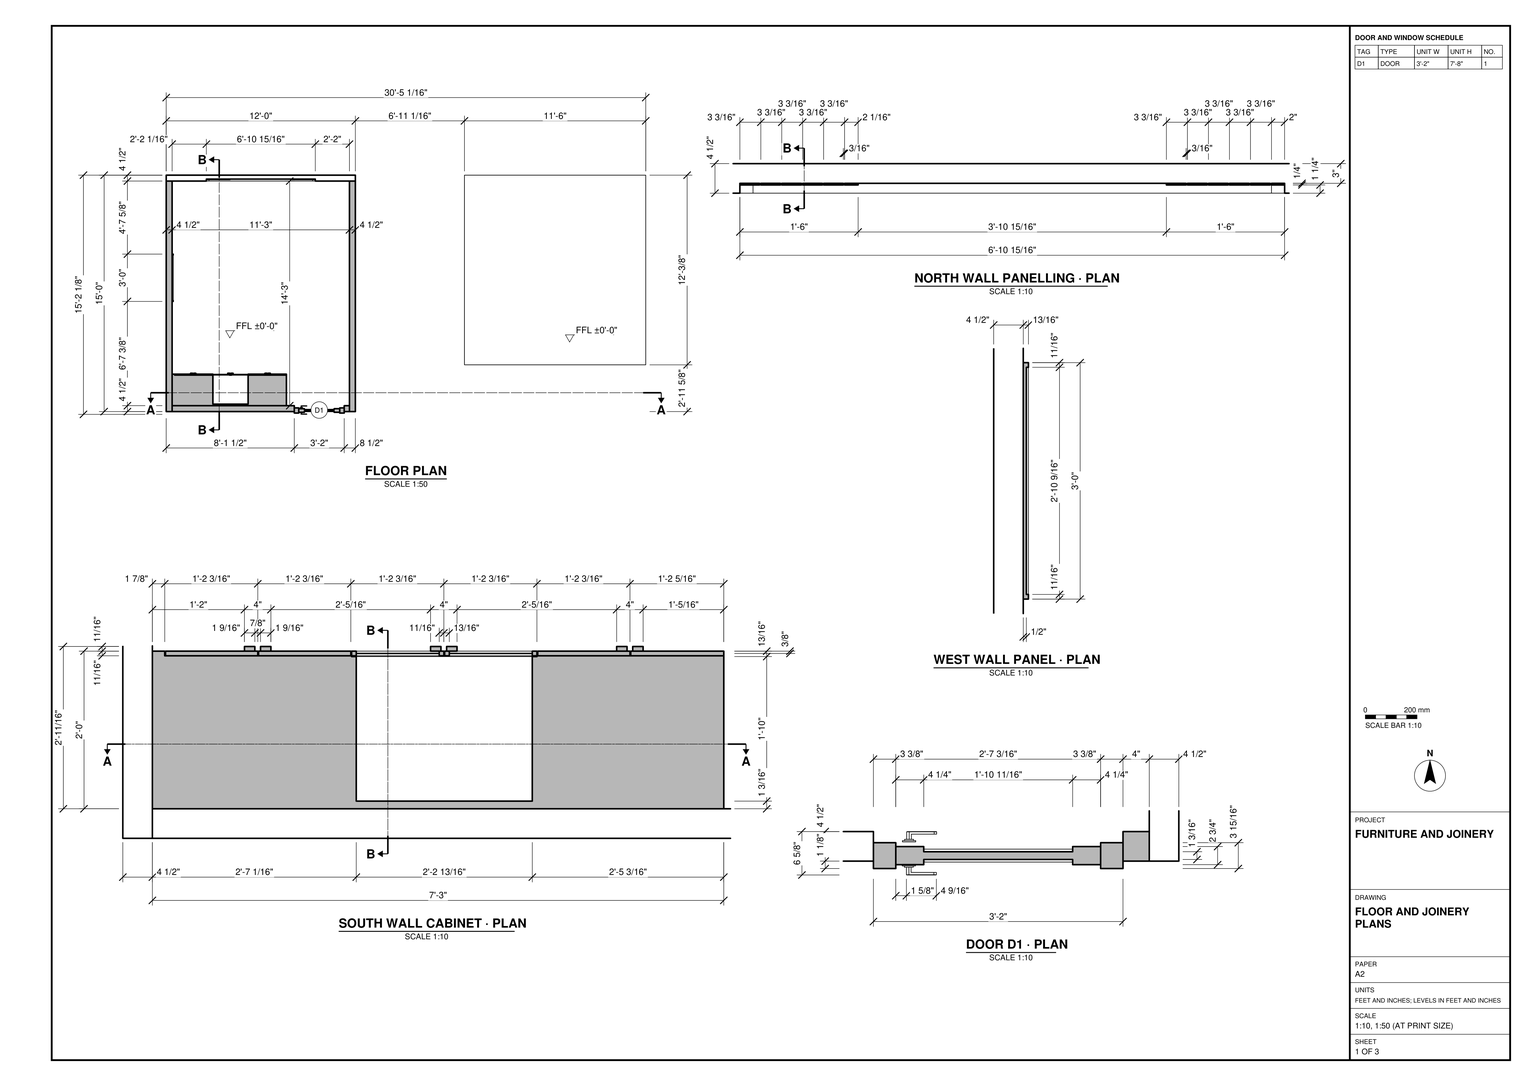
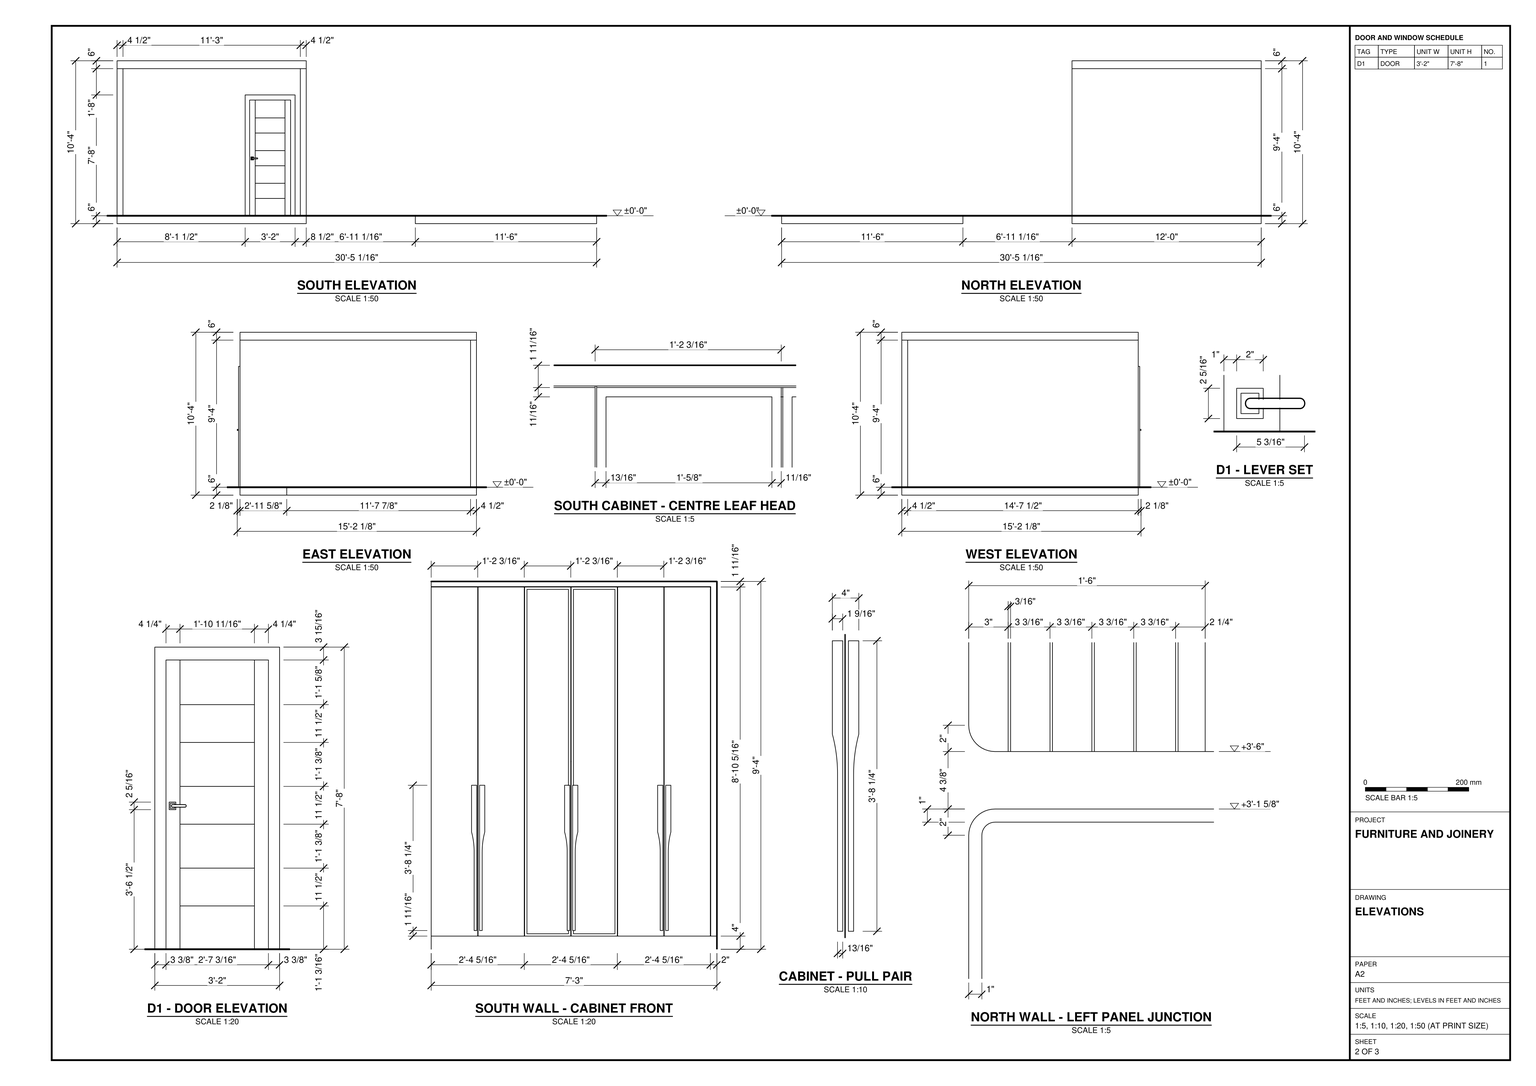
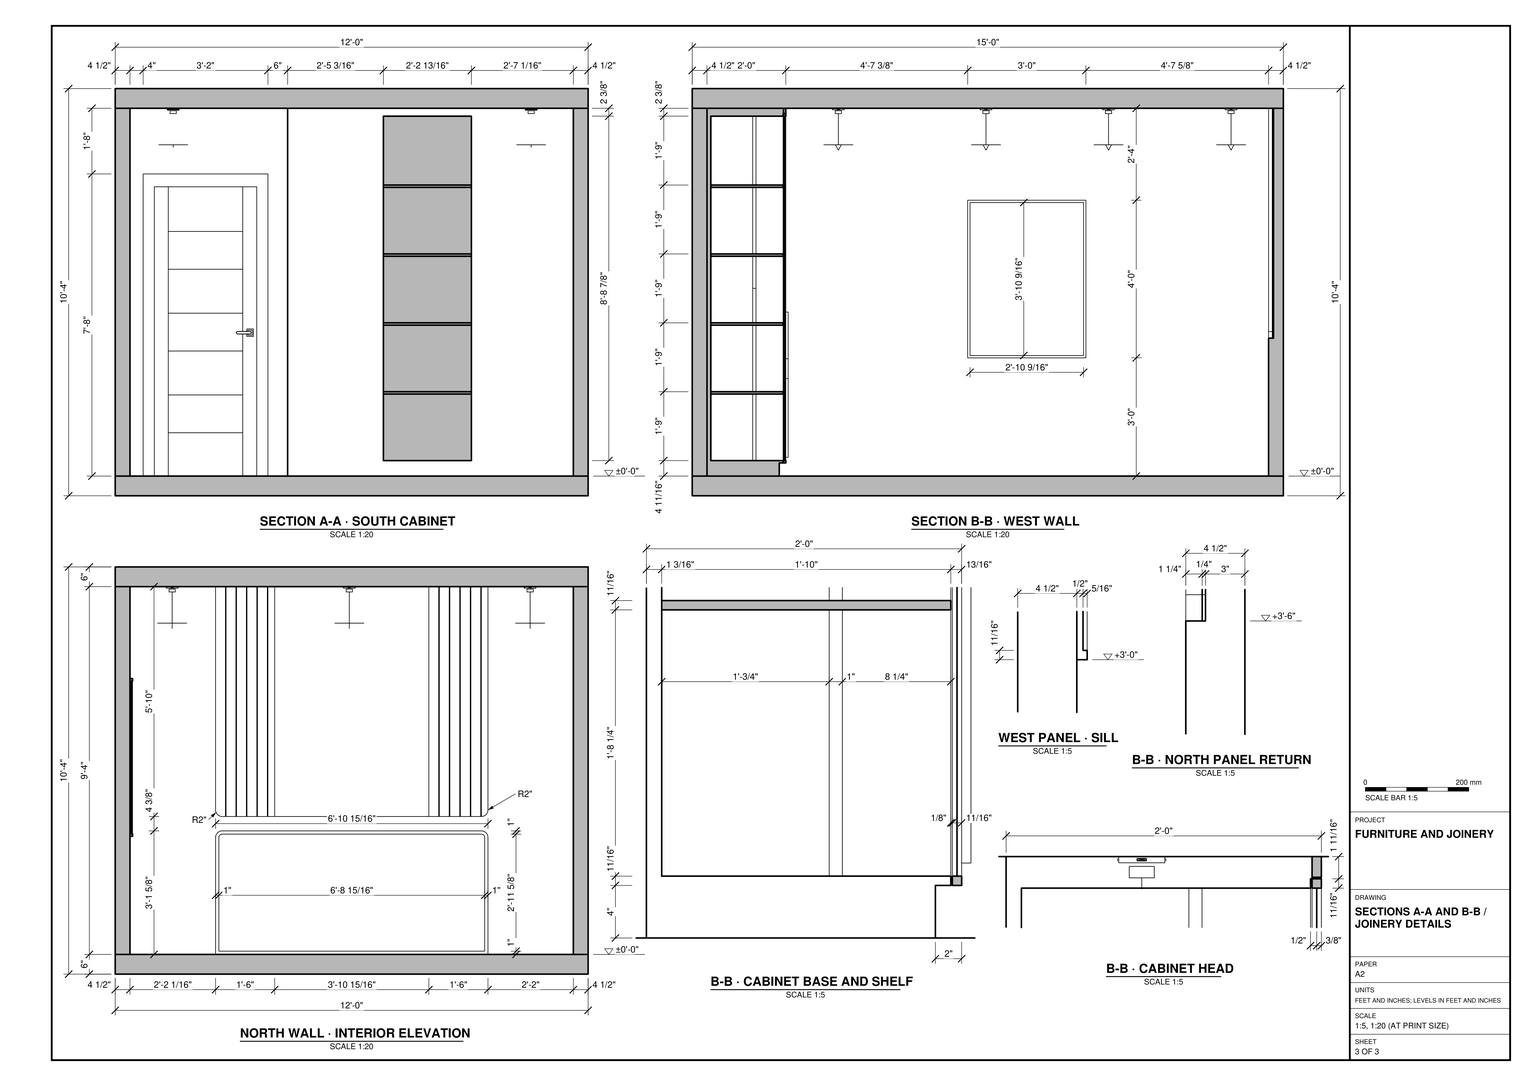
Build the room and its fitted joinery in SketchUp from task_files/diagram_01.pdf. Work in feet and inches. The complete layout is 30'-5 1/16" east to west by 15'-2 1/8" north to south, with an overall height of 10'-4". Use ±0'-0" as the finished floor level for both the room and the separate rectangular slab to its east. Keep the gap between them shown on the floor plan.

Form the room with 4 1/2" walls, a floor slab and a flat ceiling slab. Fit the framed door near the east end of the south wall, with the horizontal divisions and lever shown in elevation. Fit the full-height cabinet to the west of the door. Use the cabinet front and sections together to model the paired leaves, framed centre leaves, long pulls, shelves and recessed base.

On the north wall, model the lower framed panel and the upper panel with vertical divisions at its ends. Preserve the gap and rounded corners at their junction. On the west wall, fit the rectangular panel with its projecting sill. Place the ceiling lights as shown in section. Decor and loose items may be any suitable library components. Make the shell elements and each furniture or joinery piece separate groups or components, and use components for repeated parts. Save one SketchUp model as output_files/room_with_a_fitted_cabinet_and_wall_panelling.skp.

# SketchUp Ruby script. Lengths in inches.
U = 1.inch
M = Sketchup.active_model
def pt(a) = Geom::Point3d.new(a.map { |v| v * U })
def face(e, loops, mat)
  f = e.add_face(loops[0].map { |a| pt(a) })
  loops[1..].each { |l| e.add_face(l.map { |a| pt(a) }).erase! }
  f.material = f.back_material = mat if mat
  f
end
# faces: each face lists its corners as indices into pts; further lists are holes
def faces(e, pts, list, mat = nil) = list.each { |f| face(e, (f[0].is_a?(Array) ? f : [f]).map { |l| l.map { |i| pts[i] } }, mat) }
# xy, xz, yz: faces in a plane at the given z, y or x. An outline is a flat list of corners, or four numbers for a rectangle; further outlines are holes
def ring(l) = l.size == 4 ? [[l[0], l[1]], [l[2], l[1]], [l[2], l[3]], [l[0], l[3]]] : l.each_slice(2).to_a
def flat(e, list, mat, &to3) = list.each { |f| face(e, (f[0].is_a?(Array) ? f : [f]).map { |l| ring(l).map { |u, v| to3.(u, v) } }, mat) }
def xy(e, z, list, mat = nil) = flat(e, list, mat) { |x, y| [x, y, z] }
def xz(e, y, list, mat = nil) = flat(e, list, mat) { |x, z| [x, y, z] }
def yz(e, x, list, mat = nil) = flat(e, list, mat) { |y, z| [x, y, z] }
def lines(e, pts, list) = list.each { |a, b| e.add_line(pt(pts[a]), pt(pts[b])) }
# prism: a flat outline (further loops are holes) pulled along v
def prism(e, loops, v, mat = nil)
  f = face(e, loops, mat); d = Geom::Vector3d.new(v.map { |x| x * U })
  f.pushpull(f.normal.samedirection?(d) ? d.length : -d.length)
end
def box(e, o, s, mat = nil) = prism(e, [[o, [o[0] + s[0], o[1], o[2]], [o[0] + s[0], o[1] + s[1], o[2]], [o[0], o[1] + s[1], o[2]]]], [0, 0, s[2]], mat)
def at(x, y, z, deg = 0) = Geom::Transformation.translation(pt([x, y, z])) * Geom::Transformation.rotation(ORIGIN, Z_AXIS, deg.degrees)
def axes(o, x, y, z) = Geom::Transformation.new([*x, 0, *y, 0, *z, 0, *pt(o).to_a, 1])
def part(name) = M.definitions.add(name)
# library, detail: a bought-in or finely detailed component or shape, given as its bounding box
def library(name, o, s) = part(name).tap { |d| box(d.entities, o, s) }
def detail(e, o, s) = box(e.add_group.entities, o, s)
def put(e, d, t, mat = nil) = e.add_instance(d, t).tap { |i| i.material = mat if mat }
def group(e, t, mat = nil) = e.add_group.tap { |g| g.transformation = t; g.material = mat if mat }.entities
root = M.entities
M.materials.add("0897 AP 7835 CREAM CARESS").color = [247, 240, 216]
M.materials.add("2106173_041").color = [3, 2, 0]
M.materials.add("[Color A07]").color = [153, 0, 0]
M.materials.add("[Color M00]").color = [255, 255, 255]
M.materials.add("[Color M09]").color = [0, 0, 0]
M.materials.add("[Translucent Glass Gray]").color = [128, 128, 128]
M.materials["[Translucent Glass Gray]"].alpha = 0.5
M.materials.add("lz-doorbrown").color = [51, 28, 20]
M.materials.add("lz-doorhandle").color = [114, 114, 114]
c1 = part("Door lever handle")
xy(c1.entities,0,[[0,0,1.888,1.971]])
xy(c1.entities,0.197,[[[0,0,1.888,1.971],[0.307,0.321,1.58,1.65]]])
xy(c1.entities,0.394,[[[0.307,0.321,1.58,1.65],[0.954,0.632,0.96,0.632,0.96,1.339,0.954,1.339,0.868,1.328,0.782,1.292,0.709,1.236,0.653,1.162,0.617,1.077,0.605,0.985,0.617,0.894,0.653,0.808,0.709,0.735,0.782,0.678,0.868,0.643]],[0.954,0.632,0.868,0.643,0.782,0.678,0.709,0.735,0.653,0.808,0.617,0.894,0.605,0.985,0.617,1.077,0.653,1.162,0.709,1.236,0.782,1.292,0.868,1.328,0.954,1.339,0.96,1.339,0.96,0.632],[0.96,0.632,1.265,1.339]])
xy(c1.entities,1.181,[[1.265,0.632,1.265,1.339,4.506,1.339,4.592,1.328,4.677,1.292,4.751,1.236,4.807,1.162,4.842,1.077,4.854,0.985,4.842,0.894,4.807,0.808,4.751,0.735,4.677,0.678,4.592,0.643,4.506,0.632]])
xy(c1.entities,1.535,[[0.954,0.632,0.868,0.643,0.782,0.678,0.709,0.735,0.653,0.808,0.617,0.894,0.605,0.985,0.617,1.077,0.653,1.162,0.709,1.236,0.782,1.292,0.868,1.328,0.954,1.339,4.506,1.339,4.592,1.328,4.677,1.292,4.751,1.236,4.807,1.162,4.842,1.077,4.854,0.985,4.842,0.894,4.807,0.808,4.751,0.735,4.677,0.678,4.592,0.643,4.506,0.632]])
xy(c1.entities,1.575,[[0.956,0.671,0.878,0.681,0.802,0.713,0.737,0.763,0.687,0.828,0.656,0.904,0.645,0.985,0.656,1.067,0.687,1.143,0.737,1.208,0.802,1.258,0.878,1.289,0.956,1.3,4.503,1.3,4.581,1.289,4.657,1.258,4.722,1.208,4.772,1.143,4.804,1.067,4.815,0.985,4.804,0.904,4.772,0.828,4.722,0.763,4.657,0.713,4.581,0.681,4.503,0.671]])
xz(c1.entities,0,[[0,0,1.888,0.197]])
xz(c1.entities,0.321,[[0.307,0.197,1.58,0.394]])
xz(c1.entities,0.632,[[0.954,0.394,0.96,1.535],[0.96,0.394,0.96,1.535,4.506,1.535,4.506,1.181,1.265,1.181,1.265,0.394]])
xz(c1.entities,1.339,[[0.954,0.394,0.96,1.535],[0.96,0.394,1.265,0.394,1.265,1.181,4.506,1.181,4.506,1.535,0.96,1.535]])
xz(c1.entities,1.65,[[0.307,0.197,1.58,0.394]])
xz(c1.entities,1.971,[[0,0,1.888,0.197]])
yz(c1.entities,0,[[0,0,1.971,0.197]])
yz(c1.entities,0.307,[[0.321,0.197,1.65,0.394]])
yz(c1.entities,1.265,[[0.632,0.394,1.339,1.181]])
yz(c1.entities,1.58,[[0.321,0.197,1.65,0.394]])
yz(c1.entities,1.888,[[0,0,1.971,0.197]])
p = [[0.782,0.678,1.535],[0.868,0.643,1.535],[0.868,0.643,0.394],[0.782,0.678,0.394],[0.954,0.632,1.535],[0.954,0.632,0.394],
  [0.653,0.808,1.535],[0.709,0.735,1.535],[0.709,0.735,0.394],[0.653,0.808,0.394],[0.617,0.894,1.535],[0.617,0.894,0.394],
  [0.605,0.985,1.535],[0.605,0.985,0.394],[0.617,1.077,1.535],[0.617,1.077,0.394],[0.653,1.162,1.535],[0.653,1.162,0.394],
  [0.782,1.292,1.535],[0.709,1.236,1.535],[0.709,1.236,0.394],[0.782,1.292,0.394],[0.868,1.328,1.535],[0.868,1.328,0.394],
  [0.954,1.339,1.535],[0.954,1.339,0.394],[4.592,0.643,1.535],[4.506,0.632,1.535],[4.506,0.632,1.181],[4.592,0.643,1.181],
  [4.677,0.678,1.535],[4.677,0.678,1.181],[4.751,0.735,1.535],[4.751,0.735,1.181],[4.807,0.808,1.535],[4.807,0.808,1.181],
  [4.842,0.894,1.535],[4.842,0.894,1.181],[4.854,0.985,1.535],[4.854,0.985,1.181],[4.842,1.077,1.535],[4.842,1.077,1.181],
  [4.807,1.162,1.535],[4.807,1.162,1.181],[4.677,1.292,1.535],[4.751,1.236,1.535],[4.751,1.236,1.181],[4.677,1.292,1.181],
  [4.506,1.339,1.535],[4.592,1.328,1.535],[4.592,1.328,1.181],[4.506,1.339,1.181],[0.802,0.713,1.575],[0.878,0.681,1.575],
  [0.956,0.671,1.575],[0.96,0.632,1.535],[0.96,0.671,1.575],[4.503,0.671,1.575],[4.581,0.681,1.575],[4.657,0.713,1.575],
  [0.687,0.828,1.575],[0.737,0.763,1.575],[4.722,0.763,1.575],[4.772,0.828,1.575],[0.656,0.904,1.575],[4.804,0.904,1.575],
  [0.645,0.985,1.575],[4.815,0.985,1.575],[0.656,1.067,1.575],[4.804,1.067,1.575],[0.687,1.143,1.575],[0.737,1.208,1.575],
  [4.772,1.143,1.575],[4.722,1.208,1.575],[0.802,1.258,1.575],[4.657,1.258,1.575],[0.878,1.289,1.575],[0.956,1.3,1.575],
  [0.96,1.3,1.575],[0.96,1.339,1.535],[4.503,1.3,1.575],[4.581,1.289,1.575]]
faces(c1.entities,p,[[0,1,2,3],[1,4,5,2],[6,7,8,9],[7,0,3,8],[10,6,9,11],[12,10,11,13],[14,12,13,15],[16,14,15,17],
  [18,19,20,21],[19,16,17,20],[22,18,21,23],[24,22,23,25],[26,27,28,29],[30,26,29,31],[32,30,31,33],[34,32,33,35],
  [36,34,35,37],[38,36,37,39],[40,38,39,41],[42,40,41,43],[44,45,46,47],[45,42,43,46],[48,49,50,51],[49,44,47,50],
  [0,52,53,1],[1,53,54,4],[55,56,57,27],[54,56,55,4],[27,57,58,26],[26,58,59,30],[6,60,61,7],[7,61,52,0],
  [30,59,62,32],[32,62,63,34],[10,64,60,6],[34,63,65,36],[12,66,64,10],[36,65,67,38],[14,68,66,12],[38,67,69,40],
  [16,70,68,14],[19,71,70,16],[42,72,73,45],[40,69,72,42],[18,74,71,19],[45,73,75,44],[22,76,74,18],[24,77,76,22],
  [78,77,24,79],[79,48,80,78],[49,81,80,48],[44,75,81,49]])
c2 = part("door by lz")
put(c2.entities,c1,axes([9.99,-3.35,36.38],[1,0,0],[0,0,1],[0,-1,0]),"lz-doorhandle")
put(c2.entities,c1,axes([10.03,0.12,36.38],[1,0,0],[0,0,1],[0,1,0]),"lz-doorhandle")
g1 = group(c2.entities,at(5.91,0,0),"lz-doorbrown")
prism(g1,[[[35.43,0,0],[32.26,0,0],[32.26,0,75.4],[3.18,0,75.4],[3.18,0,0],[0,0,0],[0,0,78.74],[35.43,0,78.74]]],[0,-3.9375,0])
g2 = group(c2.entities,at(9.09,-0.59,0),"lz-doorbrown")
xy(g2,0,[[0,-2.76,3.97,-2.76,3.97,-2.36,25.11,-2.36,25.11,-2.76,29.08,-2.76,29.08,0,25.11,0,25.11,-0.39,3.97,-0.39,3.97,0,0,0]])
xy(g2,11.29,[[3.97,-2.36,25.11,-1.97],[3.97,-0.79,25.11,-0.39]])
xy(g2,21.14,[[3.97,-2.36,25.11,-1.97],[3.97,-0.79,25.11,-0.39]])
xy(g2,32.6,[[3.97,-2.36,25.11,-1.97],[3.97,-0.79,25.11,-0.39]])
xy(g2,42.45,[[3.97,-2.36,25.11,-1.97],[3.97,-0.79,25.11,-0.39]])
xy(g2,53.9,[[3.97,-2.36,25.11,-1.97],[3.97,-0.79,25.11,-0.39]])
xy(g2,63.75,[[3.97,-2.36,25.11,-1.97],[3.97,-0.79,25.11,-0.39]])
xy(g2,75.4,[[0,-2.76,0,0,3.97,0,3.97,-0.39,25.11,-0.39,25.11,0,29.08,0,29.08,-2.76,25.11,-2.76,25.11,-2.36,3.97,-2.36,3.97,-2.76]])
xz(g2,-2.76,[[0,0,3.97,75.4],[25.11,0,29.08,75.4]])
xz(g2,-2.36,[[3.97,0,25.11,11.29],[3.97,21.14,25.11,32.6],[3.97,42.45,25.11,53.9],[3.97,63.75,25.11,75.4]])
xz(g2,-1.97,[[3.97,11.29,25.11,21.14],[3.97,32.6,25.11,42.45],[3.97,53.9,25.11,63.75]])
xz(g2,-0.79,[[3.97,11.29,25.11,21.14],[3.97,32.6,25.11,42.45],[3.97,53.9,25.11,63.75]])
xz(g2,-0.39,[[3.97,0,25.11,11.29],[3.97,21.14,25.11,32.6],[3.97,42.45,25.11,53.9],[3.97,63.75,25.11,75.4]])
xz(g2,0,[[0,0,3.97,75.4],[25.11,0,29.08,75.4]])
yz(g2,0,[[-2.76,0,0,75.4]])
yz(g2,3.97,[[-2.76,0,-2.76,75.4,-2.36,75.4,-2.36,63.75,-1.97,63.75,-1.97,53.9,-2.36,53.9,-2.36,42.45,-1.97,42.45,-1.97,32.6,-2.36,32.6,-2.36,21.14,-1.97,21.14,-1.97,11.29,-2.36,11.29,-2.36,0],[-0.39,0,-0.39,11.29,-0.79,11.29,-0.79,21.14,-0.39,21.14,-0.39,32.6,-0.79,32.6,-0.79,42.45,-0.39,42.45,-0.39,53.9,-0.79,53.9,-0.79,63.75,-0.39,63.75,-0.39,75.4,0,75.4,0,0]])
yz(g2,25.11,[[-2.76,0,-2.36,0,-2.36,11.29,-1.97,11.29,-1.97,21.14,-2.36,21.14,-2.36,32.6,-1.97,32.6,-1.97,42.45,-2.36,42.45,-2.36,53.9,-1.97,53.9,-1.97,63.75,-2.36,63.75,-2.36,75.4,-2.76,75.4],[-0.39,0,0,0,0,75.4,-0.39,75.4,-0.39,63.75,-0.79,63.75,-0.79,53.9,-0.39,53.9,-0.39,42.45,-0.79,42.45,-0.79,32.6,-0.39,32.6,-0.39,21.14,-0.79,21.14,-0.79,11.29,-0.39,11.29]])
yz(g2,29.08,[[-2.76,0,0,75.4]])
c3 = part("Group140\#1")
p = [[0,0,0],[0,0,-16.35],[-0.08,0,-16.35],[0.5,-52.44,0],[-0.5,-52.44,0],[0.5,52.44,0],
  [0.5,0,0],[-0.5,52.44,0],[0.08,0,-16.35],[-0.5,0,0],[0,0,-26.47]]
lines(c3.entities,p,[[0,1],[1,2],[3,4],[5,6],[7,5],[1,8],[9,0],[0,6],[8,10],[4,9],[6,3],[2,10],
  [9,7]])
c4 = part("Rectangle Light")
put(c4.entities,c3,at(0,0,0))
c5 = part("Group\#19")
prism(c5.entities,[[[26.8,22.01,-0.71],[26.8,0,-0.71],[0,0,-0.71],[0,22.01,-0.71],[12.63,22.01,-0.71],[13.34,22.01,-0.71],[13.46,22.01,-0.71],[14.17,22.01,-0.71]]],[0,0,0.71])
c6 = part("Group94\#1")
box(c6.entities,[-9,-35,0],[3,70,0.25])
c7 = part("Group95\#1")
box(c7.entities,[-5.8,-35,0],[3,70,0.25])
c8 = part("Group96\#1")
box(c8.entities,[-2.6,-35,0],[3,70,0.25])
c9 = part("Group97\#1")
box(c9.entities,[0.6,-35,0],[3,70,0.25])
c10 = part("Group98\#1")
box(c10.entities,[3.8,-35,0],[3,70,0.25])
c11 = part("Group99\#1")
xy(c11.entities,0,[[7,-35,7,35,9,35,9,-33,8.98,-33.26,8.93,-33.52,8.85,-33.77,8.73,-34,8.59,-34.22,8.41,-34.41,8.22,-34.59,8,-34.73,7.77,-34.85,7.52,-34.93,7.26,-34.98]])
xy(c11.entities,0.25,[[7,-35,7.26,-34.98,7.52,-34.93,7.77,-34.85,8,-34.73,8.22,-34.59,8.41,-34.41,8.59,-34.22,8.73,-34,8.85,-33.77,8.93,-33.52,8.98,-33.26,9,-33,9,35,7,35]])
yz(c11.entities,7,[[-35,0,35,0.25]])
c12 = part("Group92\#1")
put(c12.entities,c6,at(0,0,0))
put(c12.entities,c7,at(0,0,0))
put(c12.entities,c8,at(0,0,0))
put(c12.entities,c9,at(0,0,0))
put(c12.entities,c10,at(0,0,0))
put(c12.entities,c11,at(0,0,0))
c13 = part("Group101\#1")
xy(c13.entities,0,[[-7,-35,-7.26,-34.98,-7.52,-34.93,-7.77,-34.85,-8,-34.73,-8.22,-34.59,-8.41,-34.41,-8.59,-34.22,-8.73,-34,-8.85,-33.77,-8.93,-33.52,-8.98,-33.26,-9,-33,-9,35,-6,35,-6,-35]])
xy(c13.entities,0.25,[[-7,-35,-6,-35,-6,35,-9,35,-9,-33,-8.98,-33.26,-8.93,-33.52,-8.85,-33.77,-8.73,-34,-8.59,-34.22,-8.41,-34.41,-8.22,-34.59,-8,-34.73,-7.77,-34.85,-7.52,-34.93,-7.26,-34.98]])
xz(c13.entities,35,[[-9,0,-6,0.25]])
yz(c13.entities,-9,[[-33,0,35,0.25]])
yz(c13.entities,-6,[[-35,0,35,0.25]])
c14 = part("Group102\#1")
box(c14.entities,[-5.8125,-35,0],[3,70,0.25])
c15 = part("Group103\#1")
box(c15.entities,[-2.625,-35,0],[3,70,0.25])
c16 = part("Group104\#1")
box(c16.entities,[0.5625,-35,0],[3,70,0.25])
c17 = part("Group105\#1")
box(c17.entities,[3.75,-35,0],[3,70,0.25])
c18 = part("Group106\#1")
xy(c18.entities,0,[[6.9375,-35,9,35]])
xy(c18.entities,0.25,[[6.9375,-35,9,35]])
yz(c18.entities,6.9375,[[-35,0,35,0.25]])
c19 = part("Group99\#2")
xz(c19.entities,35,[[6.9375,0,9,0.25]])
yz(c19.entities,9,[[-35,0,35,0.25]])
put(c19.entities,c13,at(0,0,0))
put(c19.entities,c14,at(0,0,0))
put(c19.entities,c15,at(0,0,0))
put(c19.entities,c16,at(0,0,0))
put(c19.entities,c17,at(0,0,0))
put(c19.entities,c18,at(0,0,0))
c20 = part("Group\#22")
prism(c20.entities,[[[0,0,44.23],[0,0,0],[0.79,0,0],[0.79,0,24],[0.8,0,24.51],[0.8125,0,25.02],[0.84,0,25.52],[0.88,0,26.03],[0.93,0,26.53],[0.99,0,27.04],[1.0625,0,27.54],[1.14,0,28.04],[1.24,0,28.54],[1.34,0,29.04],[1.46,0,29.53],[1.58,0,30.03],[1.58,0,44.23]]],[0,0.71,0])
c21 = part("Group\#27")
prism(c21.entities,[[[0,0,44.23],[0,0,0],[0.79,0,0],[0.79,0,24],[0.8,0,24.51],[0.8125,0,25.02],[0.84,0,25.52],[0.88,0,26.03],[0.93,0,26.53],[0.99,0,27.04],[1.0625,0,27.54],[1.14,0,28.04],[1.24,0,28.54],[1.34,0,29.04],[1.46,0,29.53],[1.58,0,30.03],[1.58,0,44.23]]],[0,0.71,0])
c22 = library("Group\#26",[-0.5,-0.5,-0.1],[96,108,0.2])
c23 = library("Group\#23",[0,0,0],[8.9,8.9,12.75])
put(root,c2,axes([91.16,4.92,6],[1.07244,0,0],[0,1,0],[0,0,1.1684]))
g3 = group(root,at(0,38.11,0))
box(g3,[0,-36,0],[144,180,6])
g4 = group(root,at(139.5,38.11,6))
xy(g4,0,[[0,-36,4.5,139.5]])
xy(g4,112,[[0,-36,4.5,139.5]],"0897 AP 7835 CREAM CARESS")
xz(g4,-36,[[0,0,4.5,112]])
xz(g4,139.5,[[0,0,4.5,112]])
yz(g4,0,[[-36,0,139.5,112]],"[Color M00]")
yz(g4,4.5,[[-36,0,139.5,112]])
g5 = group(g4,at(-135,-31.5,0))
xy(g5,0,[[0,0,87,22]])
xy(g5,4,[[0,22,0,24,1.88,24,1.88,23.29,2,23.29,2,22],[2,22,2,23.29,30.33,23.29,30.33,23.17,58.55,23.17,58.55,23.29,87,23.29,87,22],[2,23.29,16.05,24],[16.17,23.29,30.22,24],[58.67,23.29,72.72,24],
  [72.83,23.29,87,24]])
xy(g5,4,[[30.33,23.29,44.38,24],[44.5,23.29,58.55,24]],"[Color M09]")
xy(g5,4.71,[[31.04,23.29,43.67,23.65],[45.21,23.29,57.84,23.65],[31.04,23.65,43.67,24],[45.21,23.65,57.84,24]],"[Color M09]")
xy(g5,109.6,[[31.04,1.17,57.84,23.17]],"[Color A07]")
xy(g5,109.6,[[31.04,23.29,43.67,23.65],[45.21,23.29,57.84,23.65],[31.04,23.65,43.67,24],[45.21,23.65,57.84,24]],"[Color M09]")
xy(g5,110.31,[[30.33,23.17,58.55,23.29],[2,23.29,16.05,24],[16.17,23.29,30.22,24],[58.67,23.29,72.72,24],[72.83,23.29,87,24]])
xy(g5,110.31,[[30.33,23.29,44.38,24],[44.5,23.29,58.55,24]],"[Color M09]")
xy(g5,110.43,[[1.88,23.29,2,24],[2,23.29,16.05,24],[16.05,23.29,16.17,24],[16.17,23.29,30.22,24],[30.22,23.29,30.33,24],
  [30.33,23.29,58.55,24],[58.55,23.29,58.67,24],[58.67,23.29,72.72,24],[72.72,23.29,72.83,24],[72.83,23.29,87,24]])
xy(g5,112,[[0,0,87,23.29],[0,23.29,87,24]])
xz(g5,0,[[0,0,87,112]])
xz(g5,1.17,[[31.04,4.71,57.84,109.6]],"[Color A07]")
xz(g5,22,[[0,0,87,4]])
xz(g5,23.17,[[30.33,4,43.67,4.71],[43.67,4,44.38,4.71],[44.38,4,44.5,4.71],[44.5,4,45.21,4.71],[45.21,4,58.55,4.71],
  [43.67,109.6,44.38,110.31],[44.38,109.6,44.5,110.31]])
xz(g5,23.17,[[30.33,4.71,31.04,109.6],[57.84,4.71,58.55,109.6],[30.33,109.6,43.67,110.31],[44.5,109.6,45.21,110.31],[45.21,109.6,58.55,110.31]],"[Color A07]")
xz(g5,23.29,[[1.88,4,2,110.43],[2,4,16.05,110.31],[16.05,4,16.17,110.43],[16.17,4,30.22,110.31],[30.22,4,30.33,110.43],
  [30.33,4,43.67,4.71],[45.21,4,58.55,4.71],[58.55,4,58.67,110.43],[58.67,4,72.72,110.31],[72.72,4,72.83,110.43],
  [72.83,4,87,110.31],[57.84,4.71,58.55,109.6],[45.21,109.6,58.55,110.31],[2,110.31,16.05,110.43],[16.17,110.31,30.22,110.43],
  [30.33,110.31,58.55,110.43],[58.67,110.31,72.72,110.43],[72.83,110.31,87,110.43],[0,110.43,87,112]])
xz(g5,23.29,[[43.67,4,44.38,110.31],[44.5,4,45.21,110.31],[30.33,4.71,31.04,109.6],[30.33,109.6,43.67,110.31]],"[Color M09]")
xz(g5,23.65,[[31.04,4.71,43.67,109.6],[45.21,4.71,57.84,109.6]],"[Translucent Glass Gray]")
xz(g5,24,[[0,4,0,112,87,112,87,110.43,1.88,110.43,1.88,4],[2,4,16.05,110.31],[16.17,4,30.22,110.31],[58.67,4,72.72,110.31],[72.83,4,87,110.31]])
xz(g5,24,[[[30.33,4,44.38,110.31],[31.04,4.71,43.67,109.6]],[[44.5,4,58.55,110.31],[45.21,4.71,57.84,109.6]]],"[Color M09]")
yz(g5,0,[[0,0,0,112,23.29,112,23.29,110.43,24,110.43,24,4,22,4,22,0],[23.29,110.43,24,112]])
yz(g5,1.88,[[23.29,4,24,110.43]])
yz(g5,2,[[23.29,4,24,110.31]])
yz(g5,16.05,[[23.29,4,24,110.31]])
yz(g5,16.17,[[23.29,4,24,110.31]])
yz(g5,30.22,[[23.29,4,24,110.31]])
yz(g5,30.33,[[23.17,4,23.29,110.31]])
yz(g5,30.33,[[23.29,4,24,110.31]],"[Color M09]")
yz(g5,31.04,[[1.17,4.71,23.17,109.6]],"[Color A07]")
yz(g5,31.04,[[23.29,4.71,23.65,109.6],[23.65,4.71,24,109.6]],"[Color M09]")
yz(g5,43.67,[[23.29,4.71,23.65,109.6],[23.65,4.71,24,109.6]],"[Color M09]")
yz(g5,44.38,[[23.29,4,24,110.31]],"[Color M09]")
yz(g5,44.5,[[23.29,4,24,110.31]],"[Color M09]")
yz(g5,45.21,[[23.29,4.71,23.65,109.6],[23.65,4.71,24,109.6]],"[Color M09]")
yz(g5,57.84,[[1.17,4.71,23.17,109.6]],"[Color A07]")
yz(g5,57.84,[[23.29,4.71,23.65,109.6],[23.65,4.71,24,109.6]],"[Color M09]")
yz(g5,58.55,[[23.17,4,23.29,110.31]])
yz(g5,58.55,[[23.29,4,24,110.31]],"[Color M09]")
yz(g5,58.67,[[23.29,4,24,110.31]])
yz(g5,72.72,[[23.29,4,24,110.31]])
yz(g5,72.83,[[23.29,4,24,110.31]])
yz(g5,87,[[0,0,22,0,22,4,23.29,4,23.29,112,0,112],[23.29,4,24,110.31],[23.29,110.43,24,112]])
put(g5,c4,axes([57.83,14.42,57.15],[0,1,0],[0,0,-1],[1,0,0]))
put(g5,c4,axes([31.04,14.42,57.15],[0,1,0],[0,0,-1],[-1,0,0]))
g6 = group(g5,at(31.04,1.17,4.71),"[Color A07]")
xy(g6,0,[[0,0,26.8,22.01]])
put(g5,c5,at(31.04,1.17,25.6875),"[Color A07]")
put(g5,c5,at(31.04,1.17,46.66),"[Color A07]")
put(g5,c5,at(31.04,1.17,67.64),"[Color A07]")
put(g5,c5,at(31.04,1.17,88.62),"[Color A07]")
g7 = group(root,at(0,38.11,6))
xy(g7,0,[[0,-36,4.5,139.5]])
xy(g7,112,[[0,-36,4.5,139.5]])
xz(g7,-36,[[0,0,4.5,112]])
xz(g7,139.5,[[0,0,4.5,112]])
yz(g7,0,[[-36,0,139.5,112]])
yz(g7,4.5,[[-36,0,139.5,112]],"[Color M00]")
g8 = group(root,at(0,177.61,6),"0897 AP 7835 CREAM CARESS")
xy(g8,0,[[0,0,144,4.5]])
xy(g8,42,[[32.5625,0,111.5,1.5]],"0897 AP 7835 CREAM CARESS")
xy(g8,112,[[0,0,30.5625,0,30.5625,1.5,113.5,1.5,113.5,0,144,0,144,4.5,0,4.5]])
xz(g8,0,[[0,0,30.5625,0,30.5625,35.625,30.58,35.89,30.63,36.14,30.71,36.39,30.83,36.625,30.98,36.84,31.15,37.04,31.34,37.21,31.5625,37.36,31.8,37.47,32.04,37.56,32.3,37.61,32.5625,37.625,111.5,37.625,111.76,37.61,112.02,37.56,112.27,37.47,112.5,37.36,112.72,37.21,112.91,37.04,113.09,36.84,113.23,36.625,113.35,36.39,113.43,36.14,113.48,35.89,113.5,35.625,113.5,0,144,0,144,112,113.5,112,113.5,44,113.48,43.74,113.43,43.48,113.35,43.23,113.23,43,113.09,42.78,112.91,42.59,112.72,42.41,112.5,42.27,112.27,42.15,112.02,42.07,111.76,42.02,111.5,42,32.5625,42,32.3,42.02,32.04,42.07,31.8,42.15,31.5625,42.27,31.34,42.41,31.15,42.59,30.98,42.78,30.83,43,30.71,43.23,30.63,43.48,30.58,43.74,30.5625,44,30.5625,112,0,112],[31.5625,1,112.5,1,112.5,35.625,112.49,35.76,112.47,35.88,112.42,36.01,112.37,36.125,112.29,36.23,112.21,36.33,112.11,36.42,112,36.49,111.88,36.55,111.76,36.59,111.63,36.62,111.5,36.625,32.5625,36.625,32.43,36.62,32.3,36.59,32.18,36.55,32.0625,36.49,31.95,36.42,31.86,36.33,31.77,36.23,31.7,36.125,31.64,36.01,31.6,35.88,31.57,35.76,31.5625,35.625]])
xz(g8,1.5,[[48.5625,42,95.5,112]])
xz(g8,4.5,[[0,0,144,112]])
yz(g8,0,[[0,0,4.5,112]])
yz(g8,30.5625,[[0,44,1.5,112]],"0897 AP 7835 CREAM CARESS")
yz(g8,113.5,[[0,44,1.5,112]],"0897 AP 7835 CREAM CARESS")
yz(g8,144,[[0,0,4.5,112]])
p = [[32.04,0,42.07],[32.3,0,42.02],[32.3,1.5,42.02],[32.04,1.5,42.07],[32.5625,0,42],[32.5625,1.5,42],
  [111.5,0,42],[111.76,0,42.02],[111.76,1.5,42.02],[111.5,1.5,42],[112.02,0,42.07],[112.02,1.5,42.07],
  [31.8,0,42.15],[31.8,1.5,42.15],[112.27,0,42.15],[112.27,1.5,42.15],[31.5625,0,42.27],[31.5625,1.5,42.27],
  [112.5,0,42.27],[112.5,1.5,42.27],[31.34,0,42.41],[31.34,1.5,42.41],[112.72,0,42.41],[112.72,1.5,42.41],
  [31.15,0,42.59],[31.15,1.5,42.59],[112.91,0,42.59],[112.91,1.5,42.59],[30.98,0,42.78],[30.98,1.5,42.78],
  [113.09,0,42.78],[113.09,1.5,42.78],[30.83,0,43],[30.83,1.5,43],[113.23,0,43],[113.23,1.5,43],
  [30.71,0,43.23],[30.71,1.5,43.23],[113.35,0,43.23],[113.35,1.5,43.23],[30.63,0,43.48],[30.63,1.5,43.48],
  [113.43,0,43.48],[113.43,1.5,43.48],[30.58,0,43.74],[30.58,1.5,43.74],[113.48,0,43.74],[113.48,1.5,43.74],
  [30.5625,0,44],[30.5625,1.5,44],[113.5,0,44],[113.5,1.5,44]]
faces(g8,p,[[0,1,2,3],[1,4,5,2],[12,0,3,13],[16,12,13,17],[20,16,17,21],[24,20,21,25],[28,24,25,29],[32,28,29,33],
  [36,32,33,37],[40,36,37,41],[44,40,41,45],[48,44,45,49]])
faces(g8,p,[[6,7,8,9],[7,10,11,8],[10,14,15,11],[14,18,19,15],[18,22,23,19],[22,26,27,23],[26,30,31,27],[30,34,35,31],
  [34,38,39,35],[38,42,43,39],[42,46,47,43],[46,50,51,47]],"0897 AP 7835 CREAM CARESS")
g9 = group(g8,at(30.5625,0,0))
xz(g9,0,[[[0,0,82.9375,0,82.9375,35.625,82.92,35.89,82.87,36.14,82.79,36.39,82.67,36.625,82.52,36.84,82.35,37.04,82.16,37.21,81.9375,37.36,81.7,37.47,81.46,37.56,81.2,37.61,80.9375,37.625,2,37.625,1.74,37.61,1.48,37.56,1.23,37.47,1,37.36,0.78,37.21,0.59,37.04,0.41,36.84,0.27,36.625,0.15,36.39,0.07,36.14,0.02,35.89,0,35.625],[1,1,1,35.625,1.01,35.76,1.03,35.88,1.08,36.01,1.13,36.125,1.21,36.23,1.29,36.33,1.39,36.42,1.5,36.49,1.62,36.55,1.74,36.59,1.87,36.62,2,36.625,80.9375,36.625,81.07,36.62,81.2,36.59,81.32,36.55,81.4375,36.49,81.55,36.42,81.64,36.33,81.73,36.23,81.8,36.125,81.86,36.01,81.9,35.88,81.93,35.76,81.9375,35.625,81.9375,1]]])
put(g8,c12,axes([104.5,1.5,77],[1,0,0],[0,0,1],[0,-1,0]))
put(g8,c19,axes([39.5625,1.5,77],[1,0,0],[0,0,1],[0,-1,0]))
g10 = group(root,at(4.5,85.99,42),"2106173_041")
xy(g10,0,[[0,0,0.79,36]])
xy(g10,0.71,[[0.47,0.71,0.79,35.29]])
xy(g10,47.29,[[0.47,0.71,0.79,35.29]])
xy(g10,48,[[0,0,0.79,36]])
xz(g10,0,[[0,0,0.79,48]])
xz(g10,0.71,[[0.47,0.71,0.79,47.29]])
xz(g10,35.29,[[0.47,0.71,0.79,47.29]])
xz(g10,36,[[0,0,0.79,48]])
yz(g10,0,[[0,0,36,48]])
yz(g10,0.47,[[0.71,0.71,35.29,47.29]])
yz(g10,0.79,[[[0,0,36,48],[0.71,0.71,35.29,47.29]]])
put(root,c20,at(77.63,30.61,11.7),"[Color M09]")
put(root,c21,axes([76.77,30.61,11.7],[-1,0,0],[0,1,0],[0,0,1]),"[Color M09]")
g11 = group(root,at(48.43,30.61,11.7),"[Color M09]")
prism(g11,[[[0,0,44.23],[0,0,0],[-0.79,0,0],[-0.79,0,24],[-0.8,0,24.51],[-0.8125,0,25.02],[-0.84,0,25.52],[-0.88,0,26.03],[-0.93,0,26.53],[-0.99,0,27.04],[-1.0625,0,27.54],[-1.14,0,28.04],[-1.24,0,28.54],[-1.34,0,29.04],[-1.46,0,29.53],[-1.58,0,30.03],[-1.58,0,44.23]]],[0,0.71,0])
put(root,c20,at(49.3,30.61,11.7),"[Color M09]")
put(root,c21,axes([20.1,30.61,11.7],[-1,0,0],[0,1,0],[0,0,1]),"[Color M09]")
put(root,c20,at(20.97,30.61,11.7),"[Color M09]")
g12 = group(root,at(4.5,2.11,6),"0897 AP 7835 CREAM CARESS")
prism(g12,[[[131,0,0],[135,0,0],[135,0,112],[0,0,112],[0,0,0],[93,0,0],[93,0,92],[131,0,92]]],[0,4.5,0],"[Color M00]")
g13 = group(root,at(0,38.11,118))
xy(g13,0,[[[0,-36,144,144],[4.5,-7.5,139.5,139.5]],[[4.5,-7.5,139.5,139.5],[24.5,12.5,119.5,119.5]],[25.5,13.5,118.5,118.5]])
xy(g13,6,[[0,-36,144,144]])
xz(g13,-36,[[0,0,144,6]])
xz(g13,144,[[0,0,144,6]])
yz(g13,0,[[-36,0,144,6]])
yz(g13,144,[[-36,0,144,6]])
put(g13,c22,at(24.5,12.5,0))
put(root,c23,at(17.29,42.16,105.25))
put(root,c23,at(42.86,42.16,105.25))
put(root,c23,at(68.42,42.16,105.25))
put(root,c23,at(99.36,16.91,105.25))
put(root,c23,at(66.83,161.74,105.25))
put(root,c23,at(121.89,161.74,105.25))
put(root,c23,at(12.89,161.74,105.25))
put(root,c23,at(12.89,124.43,105.25))
put(root,c23,at(121.89,124.43,105.25))
put(root,c23,at(12.89,87.12,105.25))
put(root,c23,at(121.89,87.12,105.25))
put(root,c23,at(121.89,49.8,105.25))
put(root,c23,at(12.89,12.49,105.25))
put(root,c23,at(121.89,12.49,105.25))
g14 = group(root,at(227.04,37.71,0))
box(g14,[0,0,0],[138,144.4,6])
